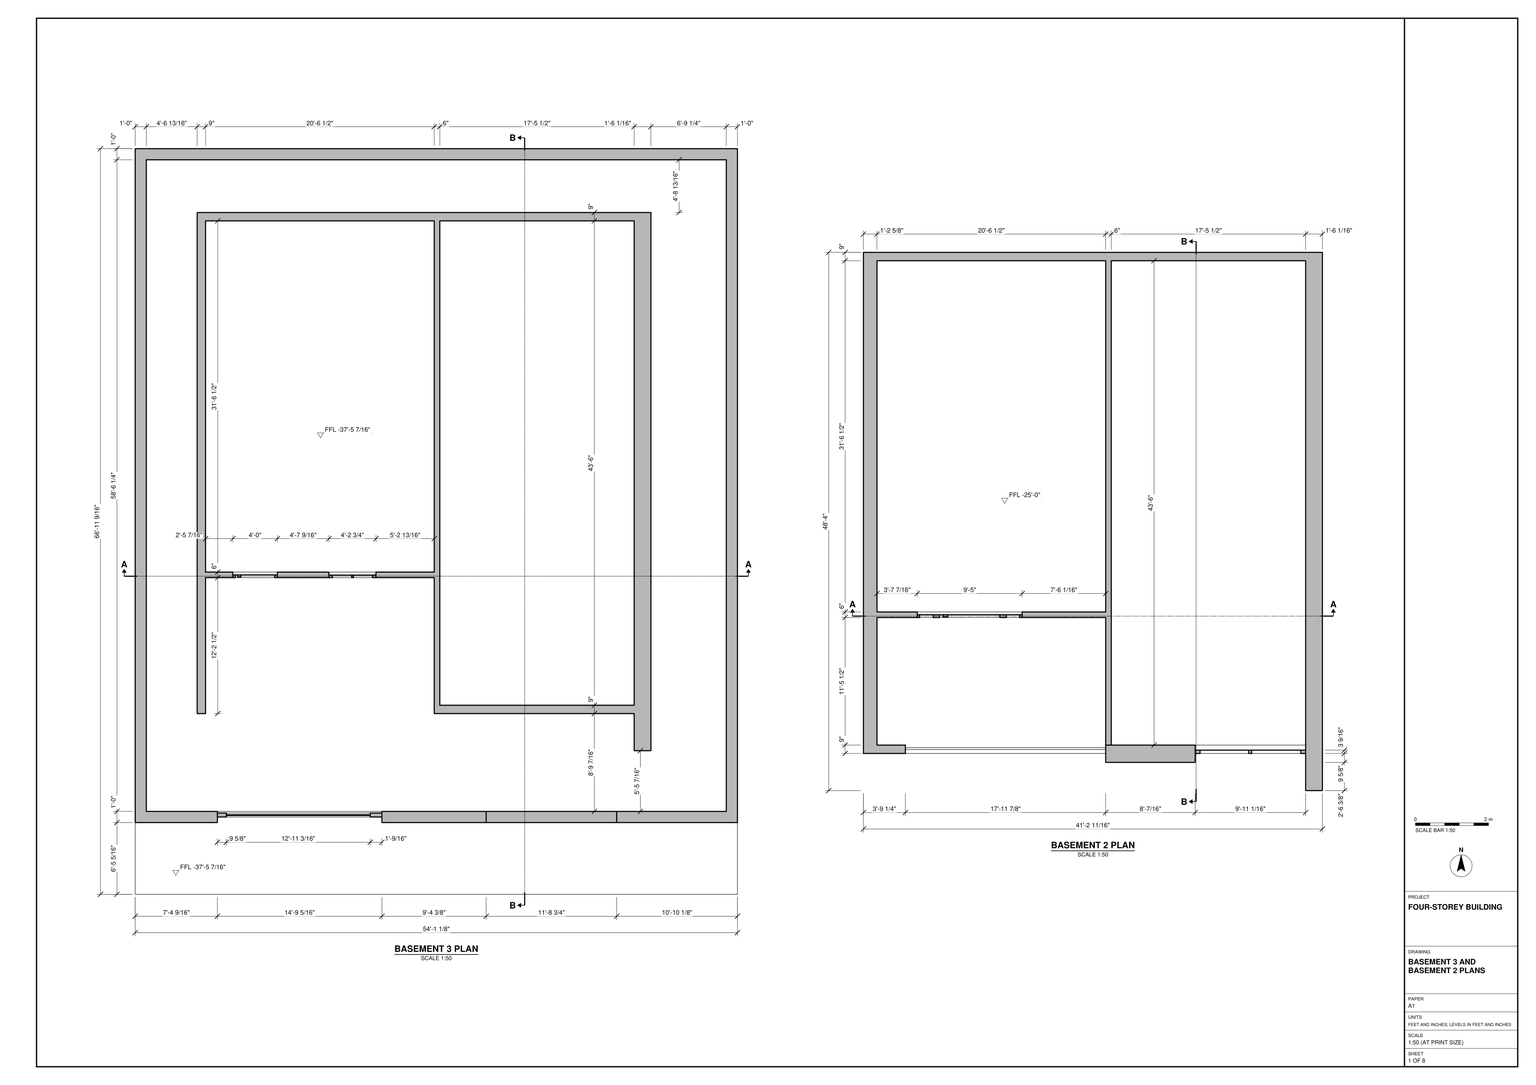
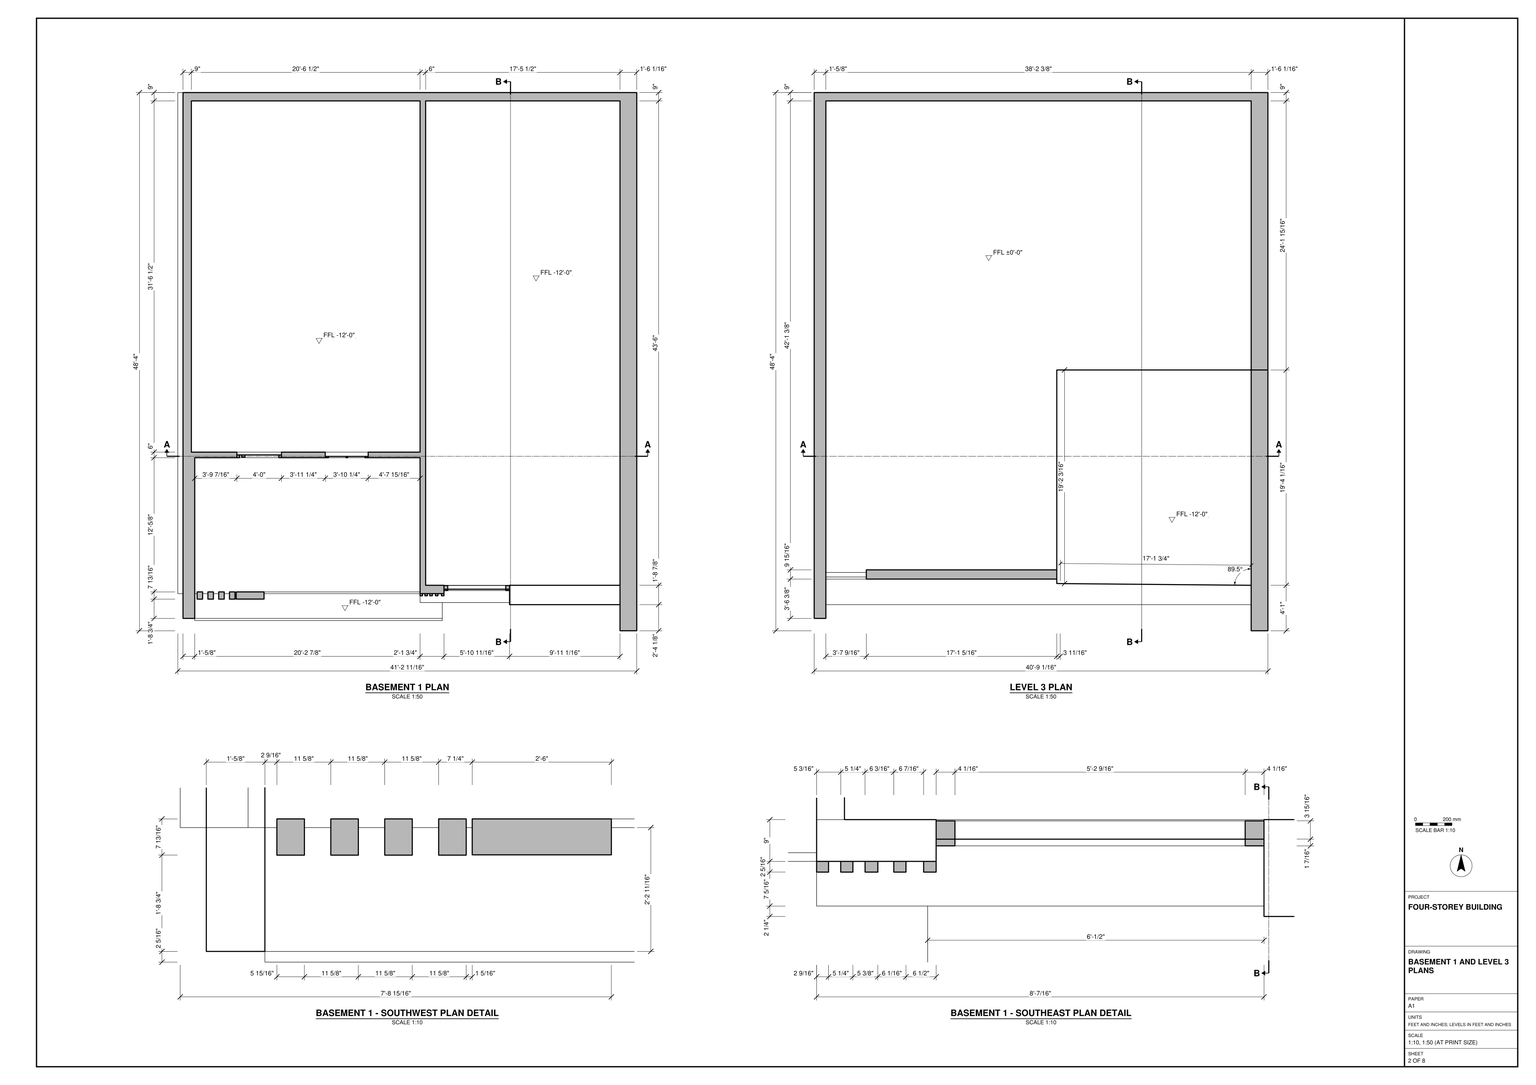
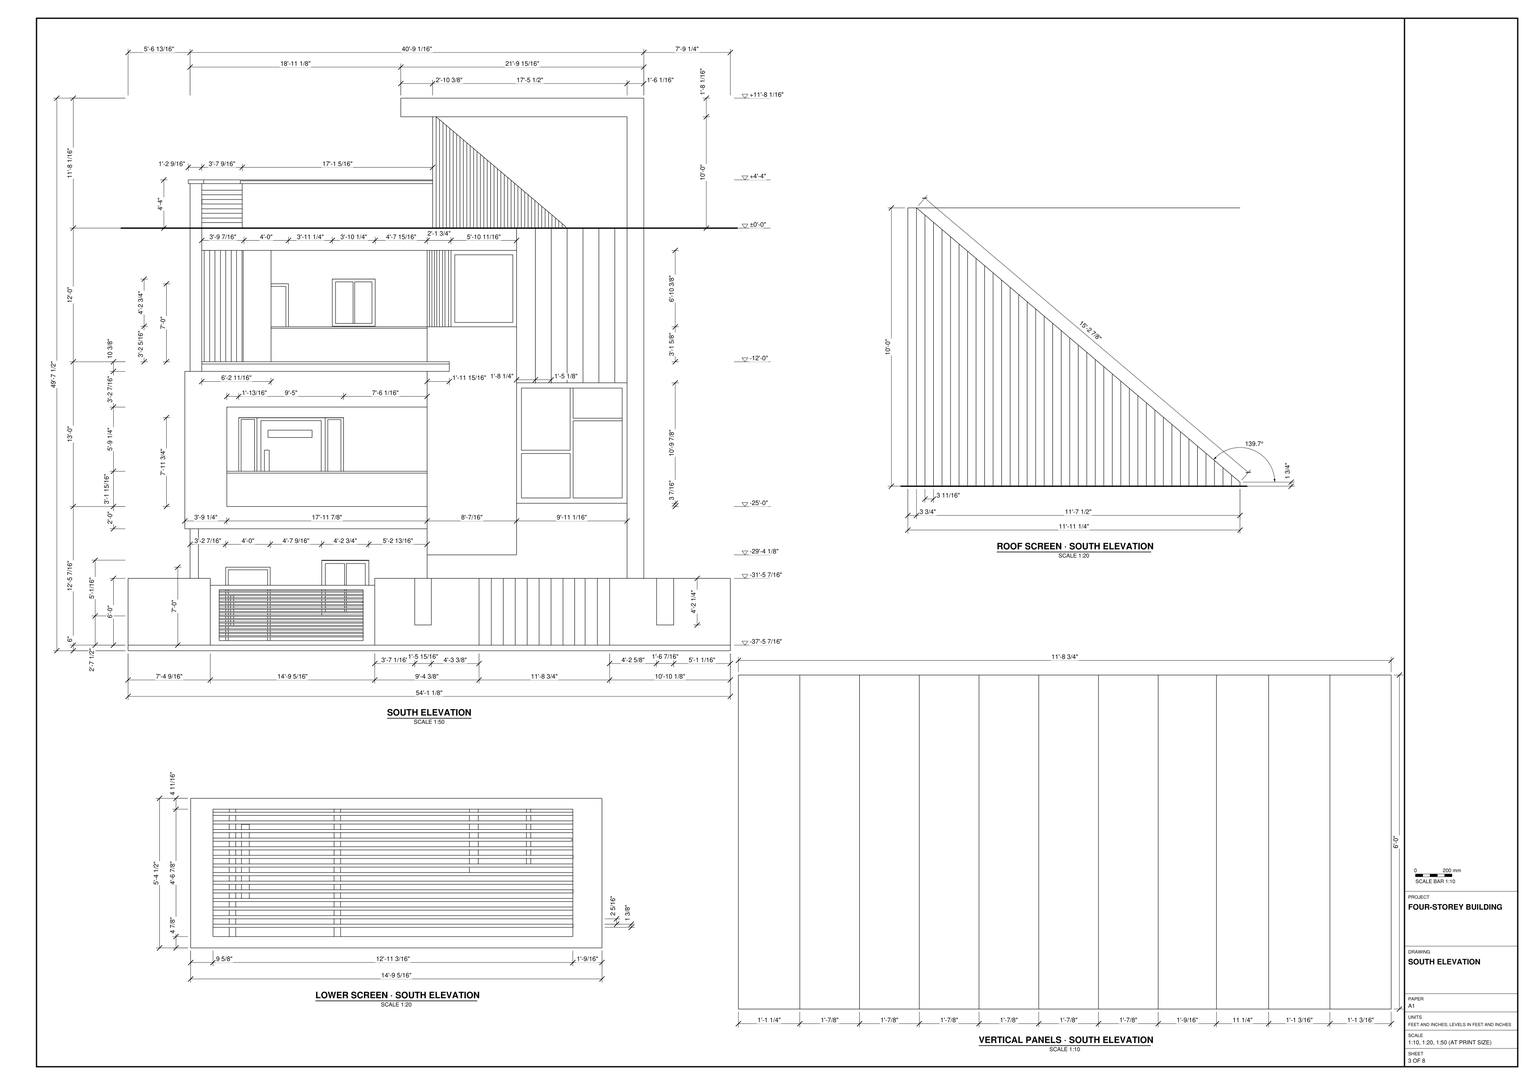
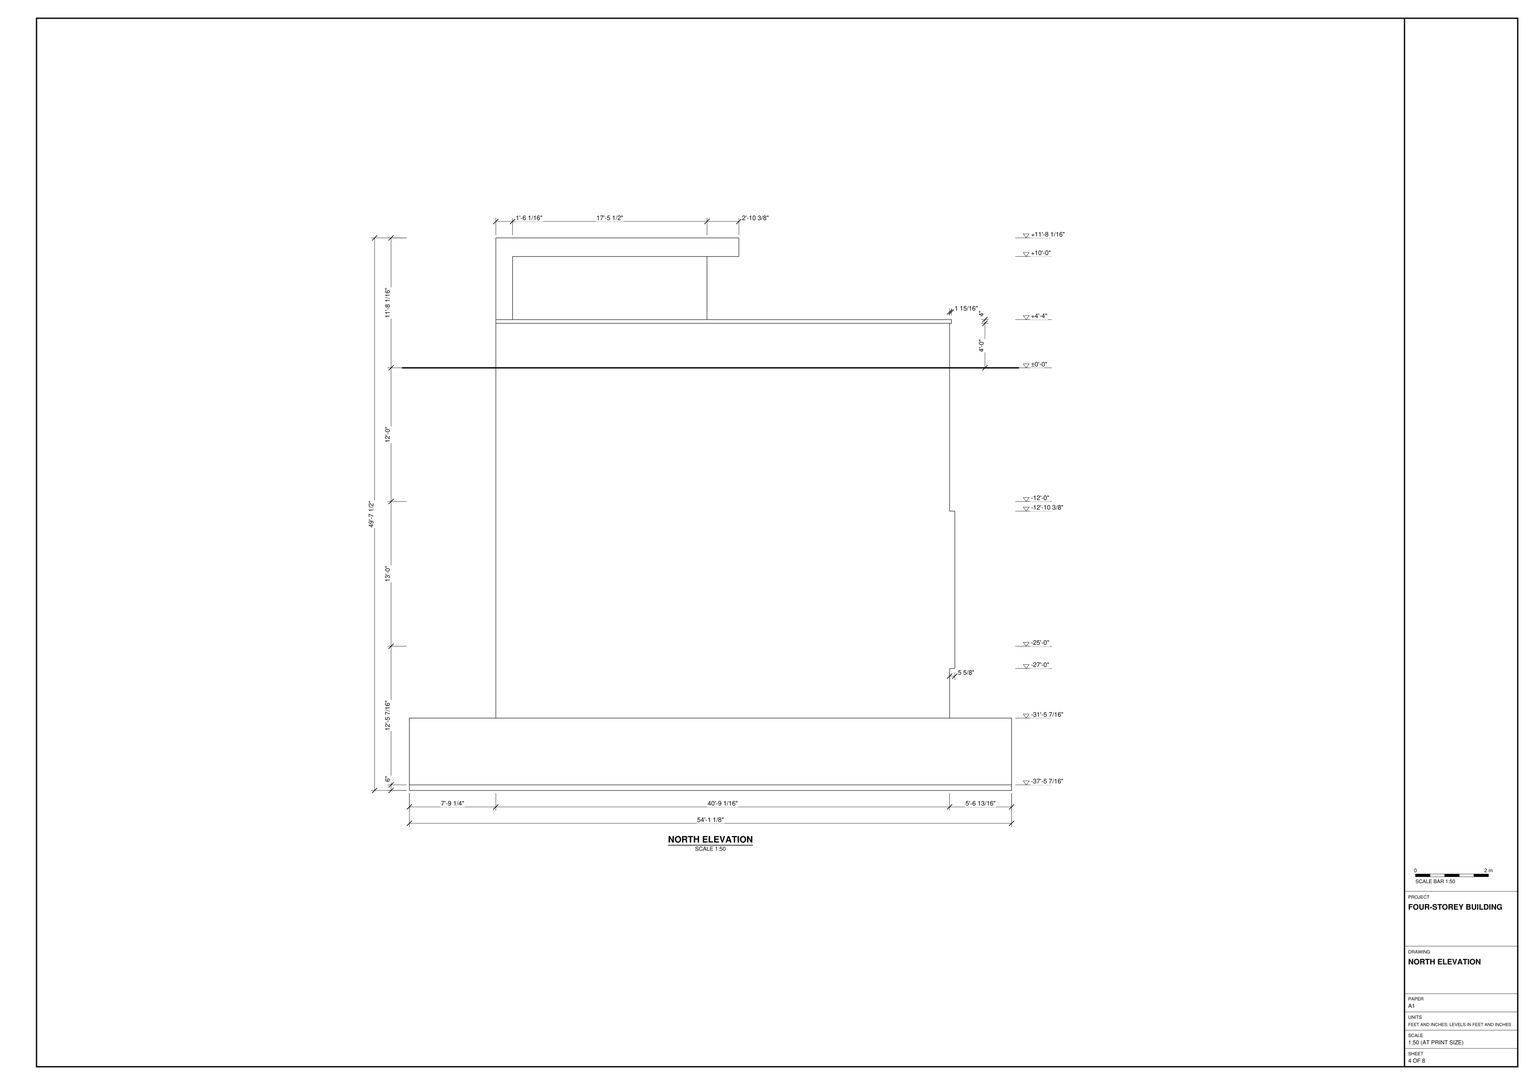
Build the four-storey building and its outer enclosure in SketchUp from task_files/diagram_01.pdf. Work in feet and inches. The complete model shall measure 69'-11 9/16" along X, 76'-9 9/16" along Y and 49'-7 1/2" along Z. Set the upper floor at ±0'-0", Basement 1 at -12'-0", Basement 2 at -25'-0" and Basement 3 at -37'-5 7/16".

Use the plans to lay out the slabs, perimeter walls and internal partitions, following the wall thicknesses and opening positions shown. Distinguish the outer enclosure at Basement 3 from the building walls inside it. Align the basement bays vertically, but follow each plan separately at the south edge, where the slab projections and recesses differ. At the upper level, preserve the southeast cutback overlooking Basement 1. Follow the sheets for stairs, built-in joinery and main furniture wherever shown.

Use the south elevation and enlarged details to model the doors, framed windows, horizontal lower screen, vertical panels and sloping roof screen beneath the raised roof frame. Decor and loose items shown may be any suitable library components. Keep shell elements such as walls, slabs and roof, and each furniture or joinery piece, in separate groups or components; use components for repeated parts. Save one SketchUp model as output_files/four_storey_building_with_a_screened_south_elevation.skp.

# SketchUp Ruby script. Lengths in inches.
U = 1.inch
M = Sketchup.active_model
def pt(a) = Geom::Point3d.new(a.map { |v| v * U })
def face(e, loops, mat)
  f = e.add_face(loops[0].map { |a| pt(a) })
  loops[1..].each { |l| e.add_face(l.map { |a| pt(a) }).erase! }
  f.material = f.back_material = mat if mat
  f
end
# faces: each face lists its corners as indices into pts; further lists are holes
def faces(e, pts, list, mat = nil) = list.each { |f| face(e, (f[0].is_a?(Array) ? f : [f]).map { |l| l.map { |i| pts[i] } }, mat) }
# xy, xz, yz: faces in a plane at the given z, y or x. An outline is a flat list of corners, or four numbers for a rectangle; further outlines are holes
def ring(l) = l.size == 4 ? [[l[0], l[1]], [l[2], l[1]], [l[2], l[3]], [l[0], l[3]]] : l.each_slice(2).to_a
def flat(e, list, mat, &to3) = list.each { |f| face(e, (f[0].is_a?(Array) ? f : [f]).map { |l| ring(l).map { |u, v| to3.(u, v) } }, mat) }
def xy(e, z, list, mat = nil) = flat(e, list, mat) { |x, y| [x, y, z] }
def xz(e, y, list, mat = nil) = flat(e, list, mat) { |x, z| [x, y, z] }
def yz(e, x, list, mat = nil) = flat(e, list, mat) { |y, z| [x, y, z] }
def lines(e, pts, list) = list.each { |a, b| e.add_line(pt(pts[a]), pt(pts[b])) }
# prism: a flat outline (further loops are holes) pulled along v
def prism(e, loops, v, mat = nil)
  f = face(e, loops, mat); d = Geom::Vector3d.new(v.map { |x| x * U })
  f.pushpull(f.normal.samedirection?(d) ? d.length : -d.length)
end
def box(e, o, s, mat = nil) = prism(e, [[o, [o[0] + s[0], o[1], o[2]], [o[0] + s[0], o[1] + s[1], o[2]], [o[0], o[1] + s[1], o[2]]]], [0, 0, s[2]], mat)
def at(x, y, z, deg = 0) = Geom::Transformation.translation(pt([x, y, z])) * Geom::Transformation.rotation(ORIGIN, Z_AXIS, deg.degrees)
def axes(o, x, y, z) = Geom::Transformation.new([*x, 0, *y, 0, *z, 0, *pt(o).to_a, 1])
def part(name) = M.definitions.add(name)
# library, detail: a bought-in or finely detailed component or shape, given as its bounding box
def library(name, o, s) = part(name).tap { |d| box(d.entities, o, s) }
def detail(e, o, s) = box(e.add_group.entities, o, s)
def put(e, d, t, mat = nil) = e.add_instance(d, t).tap { |i| i.material = mat if mat }
def group(e, t, mat = nil) = e.add_group.tap { |g| g.transformation = t; g.material = mat if mat }.entities
root = M.entities
M.materials.add("[0033_NavajoWhite]").color = [255, 222, 173]
M.materials.add("[0043_SaddleBrown]").color = [100, 69, 19]
M.materials.add("[0099_LightSteelBlue]").color = [176, 196, 222]
M.materials.add("[0134_DimGray]").color = [105, 105, 105]
M.materials.add("[Blacktop Old 01]").color = [132, 136, 139]
M.materials.add("[Color C02]").color = [255, 204, 153]
M.materials.add("[Color M04]").color = [142, 142, 142]
M.materials.add("[Color M05]").color = [114, 114, 114]
M.materials.add("[Color M06]").color = [86, 86, 86]
M.materials.add("[Concrete Aggregate Smoke]").color = [154, 150, 148]
M.materials.add("[Concrete Scored Jointless]").color = [140, 133, 127]
M.materials.add("[Metal Seamed]").color = [118, 119, 115]
M.materials.add("[Metal Silver]").color = [234, 233, 238]
M.materials.add("[Mirror 02]").color = [229, 229, 229]
M.materials.add("[Pavers with Grass Brick]").color = [187, 192, 176]
M.materials.add("[Polished Concrete Old]").color = [229, 229, 229]
M.materials.add("[Stone Brushed Khaki]").color = [226, 190, 149]
M.materials.add("[Translucent Glass Gray]").color = [128, 128, 128]
M.materials["[Translucent Glass Gray]"].alpha = 0.5
M.materials.add("[Wood Bamboo]").color = [177, 105, 43]
M.materials.add("[Wood Fence with Lattice]").color = [170, 106, 61]
M.materials.add("[Wood Floor]").color = [155, 105, 61]
c1 = part("Group\#1")
xy(c1.entities,0,[[0,0,101.9375,6.5625]],"[Wood Bamboo]")
xy(c1.entities,7.64,[[49.36,0,53.16,6.5625]])
xy(c1.entities,7.64,[[7.64,0,49.36,6.5625],[53.16,0,94.29,6.5625]],"[Wood Bamboo]")
xy(c1.entities,122.36,[[7.64,0,49.36,6.5625],[53.16,0,94.29,6.5625]],"[Wood Bamboo]")
xy(c1.entities,130,[[0,0,101.9375,6.5625]],"[Wood Bamboo]")
xz(c1.entities,0,[[[0,0,101.9375,130],[7.64,7.64,7.64,122.36,49.36,122.36,49.36,7.64,53.16,7.64,53.16,122.36,94.29,122.36,94.29,7.64]]],"[Wood Bamboo]")
xz(c1.entities,6.5625,[[7.64,7.64,49.36,122.36],[53.16,7.64,94.29,122.36]],"[Translucent Glass Gray]")
xz(c1.entities,6.5625,[[[0,0,101.9375,130],[7.64,7.64,94.29,7.64,94.29,122.36,53.16,122.36,53.16,7.64,49.36,7.64,49.36,122.36,7.64,122.36]]],"[Wood Bamboo]")
yz(c1.entities,0,[[0,0,6.5625,130]],"[Wood Bamboo]")
yz(c1.entities,7.64,[[0,7.64,6.5625,122.36]],"[Wood Bamboo]")
yz(c1.entities,49.36,[[0,7.64,6.5625,122.36]],"[Wood Bamboo]")
yz(c1.entities,53.16,[[0,7.64,6.5625,122.36]],"[Wood Bamboo]")
yz(c1.entities,94.29,[[0,7.64,6.5625,122.36]],"[Wood Bamboo]")
yz(c1.entities,101.9375,[[0,0,6.5625,130]],"[Wood Bamboo]")
c2 = part("Group\#2")
xy(c2.entities,0,[[0,0,48,3]],"[Wood Bamboo]")
xy(c2.entities,2.8,[[2.8,0,45.2,3]],"[Wood Bamboo]")
xy(c2.entities,21.03,[[5.27,0.5,8.64,3]],"[Metal Seamed]")
xy(c2.entities,53.28,[[5.27,0.5,8.64,3]],"[Metal Seamed]")
xy(c2.entities,81.2,[[2.8,0,45.2,3]],"[Wood Bamboo]")
xy(c2.entities,84,[[0,0,48,3]],"[Wood Bamboo]")
xz(c2.entities,0,[[[0,0,48,84],[2.8,2.8,45.2,81.2]]],"[Wood Bamboo]")
xz(c2.entities,0.5,[[5.27,21.03,8.64,53.28]],"[Metal Seamed]")
xz(c2.entities,3,[[[0,0,48,84],[2.8,2.8,45.2,81.2]],[[2.8,2.8,45.2,81.2],[5.27,21.03,8.64,53.28]],[5.27,21.03,8.64,53.28]],"[Wood Bamboo]")
yz(c2.entities,0,[[0,0,3,84]],"[Wood Bamboo]")
yz(c2.entities,2.8,[[0,2.8,3,81.2]],"[Wood Bamboo]")
yz(c2.entities,5.27,[[0.5,21.03,3,53.28]],"[Metal Seamed]")
yz(c2.entities,8.64,[[0.5,21.03,3,53.28]],"[Metal Seamed]")
yz(c2.entities,45.2,[[0,2.8,3,81.2]],"[Wood Bamboo]")
yz(c2.entities,48,[[0,0,3,84]],"[Wood Bamboo]")
c3 = library("Group\#3",[0,0,0],[73.75,3,84])
c4 = library("Group\#5",[0,0,0],[79.0625,3.5625,79.0625])
c5 = library("Group\#6",[0,0,0],[68.25,4.25,58.625])
xy(root,-2306.375,[[0,117.99,649.125,921.56]],"[Concrete Scored Jointless]")
xy(root,-2300.375,[[0,195.31,0,921.56,649.125,921.56,649.125,195.31,519,195.31,519,207.31,637.125,207.31,637.125,909.56,12,909.56,12,207.31,88.59,207.31,88.59,195.31],[265.91,195.31,378.28,207.31],[378.28,195.31,519,207.31],[66.8125,312.74,75.8125,459.24],[328.3125,321.74,537.8125,843.74],
  [75.8125,465.24,322.3125,843.74]])
xy(root,-2300.375,[[[12,207.31,637.125,909.56],[75.8125,465.24,322.3125,843.74],[66.8125,312.74,75.8125,459.24]]],"[Concrete Aggregate Smoke]")
xy(root,-2300.375,[[0,117.99,649.125,117.99,649.125,195.31,265.91,195.31,265.91,207.31,88.59,207.31,88.59,195.31,0,195.31]],"[Pavers with Grass Brick]")
xy(root,-2268.89,[[208.76,459.24,259.51,465.24]])
xy(root,-2228.375,[[66.8125,323.19,75.8125,459.24]],"[Color C02]")
xy(root,-2228.375,[[378.28,195.31,519,207.31]],"[Polished Concrete Old]")
xy(root,-2228.375,[[0,195.31,88.59,195.31,88.59,207.31,12,207.31,12,909.56,637.125,909.56,637.125,207.31,519,207.31,519,195.31,649.125,195.31,649.125,921.56,0,921.56],[265.91,195.31,378.28,207.31]],"[Wood Fence with Lattice]")
xy(root,-2216.375,[[105.22,459.24,153.22,465.24]])
xy(root,-2209.21,[[208.76,459.24,259.51,465.24]])
xy(root,-2203.05,[[322.3125,303.12,418.75,312.74]],"[Stone Brushed Khaki]")
xy(root,-2174.9375,[[61.1875,312.74,66.8125,323.19]])
xy(root,-2174.9375,[[61.1875,323.19,75.8125,459.24],[61.1875,459.24,66.8125,852.74]],"[Color C02]")
xy(root,-2174.9375,[[75.8125,312.74,322.3125,459.24]],"[Wood Floor]")
xy(root,-2164.25,[[75.8125,465.24,322.3125,843.74]])
xy(root,-2156.75,[[328.3125,321.74,537.8125,843.74]])
xy(root,-2150.9375,[[106.4375,316.93,322.3125,318.93],[106.4375,318.93,322.3125,318.93,322.3125,459.24,75.8125,459.24,75.8125,321.74,106.4375,321.74],[328.3125,321.74,537.8125,843.74],[119.26,459.24,232.26,465.24],[75.8125,465.24,322.3125,843.74]])
xy(root,-2150.9375,[[106.4375,312.74,322.3125,316.93]],"[Polished Concrete Old]")
xy(root,-2147.48,[[418.75,312.74,537.8125,321.74]])
xy(root,-2115,[[106.4375,316.93,322.3125,318.93]])
xy(root,-2113,[[106.4375,316.93,322.3125,318.93]],"[Metal Silver]")
xy(root,-2055.3125,[[119.26,459.24,232.26,465.24]])
xy(root,-2043.75,[[106.4375,312.74,322.3125,321.74]],"[Polished Concrete Old]")
xy(root,-2030.9375,[[75.8125,321.74,322.3125,459.24]],"[Wood Floor]")
xy(root,-2017.62,[[418.75,300.87,537.8125,321.74]])
xy(root,-2015.125,[[75.8125,465.24,322.3125,843.74]])
xy(root,-2005.3125,[[66.8125,286.06,79.4375,312.74],[322.3125,303.12,346.25,312.74]])
xy(root,-2005.3125,[[61.1875,312.74,66.8125,852.74]],"[Color C02]")
xy(root,-2005.3125,[[79.4375,286.06,79.4375,312.74,322.3125,312.74,322.3125,303.12,346.25,303.12,346.25,286.06]],"[Color M05]")
xy(root,-1999,[[328.3125,321.74,537.8125,843.74]])
xy(root,-1997.375,[[79.4375,286.06,346.25,312.74]])
xy(root,-1997.375,[[79.4375,283.74,346.25,286.06]],"[Color M05]")
xy(root,-1994.9375,[[322.3125,303.12,346.25,312.74],[82.02,306.81,87.96,312.74],[93.65,306.81,99.58,312.74],[105.27,306.81,111.21,312.74],[116.9,306.81,122.83,312.74],
  [124.125,306.87,154.125,312.74],[75.8125,312.74,79.4375,459.24],[82.02,312.74,87.96,314.62],[93.65,312.74,99.58,314.62],[105.27,312.74,111.21,314.62],
  [116.9,312.74,122.83,314.62],[124.125,312.74,154.125,314.62],[154.125,312.74,322.3125,314.62],[328.3125,321.74,537.8125,843.74],[124.9,459.24,172.9,465.24],
  [75.8125,465.24,322.3125,843.74]])
xy(root,-1994.9375,[[79.4375,283.74,346.25,286.06],[79.4375,312.74,82.02,312.74,82.02,314.62,87.96,314.62,87.96,312.74,93.65,312.74,93.65,314.62,99.58,314.62,99.58,312.74,105.27,312.74,105.27,314.62,111.21,314.62,111.21,312.74,116.9,312.74,116.9,314.62,122.83,314.62,122.83,312.74,124.125,312.74,124.125,314.62,322.3125,314.62,322.3125,459.24,79.4375,459.24]],"[Color M05]")
xy(root,-1994.9375,[[79.4375,286.06,346.25,286.06,346.25,303.12,322.3125,303.12,322.3125,312.74,154.125,312.74,154.125,306.87,124.125,306.87,124.125,312.74,122.83,312.74,122.83,306.81,116.9,306.81,116.9,312.74,111.21,312.74,111.21,306.81,105.27,306.81,105.27,312.74,99.58,312.74,99.58,306.81,93.65,306.81,93.65,312.74,87.96,312.74,87.96,306.81,82.02,306.81,82.02,312.74,79.4375,312.74]],"[Color M06]")
xy(root,-1958.9375,[[154.125,312.74,322.3125,314.62]])
xy(root,-1957.3125,[[322.3125,310.43,324.88,312.74],[327.51,310.43,330.13,312.74],[332.76,310.43,335.51,312.74],[338.95,310.43,341.57,312.74],[345.38,310.43,348.07,312.74]])
xy(root,-1957.3125,[[154.125,312.74,322.3125,314.62]],"[Metal Silver]")
xy(root,-1957.3125,[[322.3125,303.12,418.75,303.12,418.75,321.74,348.07,321.74,348.07,310.43,345.38,310.43,345.38,312.74,341.57,312.74,341.57,310.43,338.95,310.43,338.95,312.74,335.51,312.74,335.51,310.43,332.76,310.43,332.76,312.74,330.13,312.74,330.13,310.43,327.51,310.43,327.51,312.74,324.88,312.74,324.88,310.43,322.3125,310.43]],"[Stone Brushed Khaki]")
xy(root,-1956.62,[[220.125,459.24,266.375,465.24]])
xy(root,-1910.9375,[[124.9,459.24,172.9,465.24]])
xy(root,-1905.81,[[220.125,459.24,266.375,465.24]])
xy(root,-1875,[[82.02,306.81,87.96,314.62]])
xy(root,-1874.9375,[[322.3125,300.87,322.3125,310.43,324.88,310.43,324.88,312.74,327.51,312.74,327.51,310.43,330.13,310.43,330.13,312.74,332.76,312.74,332.76,310.43,335.51,310.43,335.51,312.74,338.95,312.74,338.95,310.43,341.57,310.43,341.57,312.74,345.38,312.74,345.38,310.43,348.07,310.43,348.07,321.74,418.75,321.74,418.75,300.87],[322.3125,310.43,324.88,312.74],[327.51,310.43,330.13,312.74],[332.76,310.43,335.51,312.74],[338.95,310.43,341.57,312.74],
  [345.38,310.43,348.07,312.74]])
xy(root,-1874.9375,[[[79.4375,300.87,322.3125,459.24],[124.125,306.87,154.125,314.62],[93.65,306.81,99.58,314.62],[105.27,306.81,111.21,314.62],[116.9,306.81,122.83,314.62]]],"[Wood Floor]")
xy(root,-1857.1875,[[328.3125,321.74,537.8125,843.74]])
xy(root,-1856.8125,[[75.8125,465.24,322.3125,843.74]])
xy(root,-1850.9375,[[537.8125,321.74,471.54,322.34,464.2,322.41,460.52,322.44,456.85,322.47,453.18,322.51,445.84,322.57,442.17,322.61,434.83,322.67,431.16,322.71,423.82,322.77,420.14,322.81,412.8,322.87,409.13,322.91,405.46,322.9375,401.79,322.97,398.12,323,394.45,323.04,387.11,323.1,383.4375,323.14,379.76,323.17,376.09,323.2,372.42,323.24,365.08,323.3,361.41,323.34,354.07,323.4,350.4,323.4375,346.73,323.47,343.06,323.5,339.38,323.54,332.04,323.6,328.3125,323.66,328.3125,553.79,537.8125,553.79],[123.02,328.43,328.3125,338.37],[537.8125,553.79,555.875,852.74],[79.4375,843.74,537.8125,852.74]])
xy(root,-1850.9375,[[79.4375,300.87,537.8125,300.87,537.8125,321.74,471.54,322.34,464.2,322.41,460.52,322.44,456.85,322.47,453.18,322.51,445.84,322.57,442.17,322.61,434.83,322.67,431.16,322.71,423.82,322.77,420.14,322.81,412.8,322.87,409.13,322.91,405.46,322.9375,401.79,322.97,398.12,323,394.45,323.04,387.11,323.1,383.4375,323.14,379.76,323.17,376.09,323.2,372.42,323.24,365.08,323.3,361.41,323.34,354.07,323.4,350.4,323.4375,346.73,323.47,343.06,323.5,339.38,323.54,332.04,323.6,328.3125,323.66,328.3125,328.43,79.4375,328.43]],"[0099_LightSteelBlue]")
xy(root,-1850.9375,[[79.4375,328.43,123.02,328.43,123.02,338.37,328.3125,338.37,328.3125,553.79,537.8125,553.79,537.8125,843.74,79.4375,843.74]],"[Blacktop Old 01]")
xy(root,-1844.98,[[123.02,330.7,148.02,335.57]])
xy(root,-1844.98,[[79.4375,330.7,123.02,335.57]],"[Color M05]")
xy(root,-1840.1,[[123.02,330.7,148.02,335.57]])
xy(root,-1840.1,[[79.4375,330.7,123.02,335.57]],"[Color M05]")
xy(root,-1834.98,[[123.02,330.7,148.02,335.57]])
xy(root,-1834.98,[[79.4375,330.7,123.02,335.57]],"[Color M05]")
xy(root,-1830.1,[[123.02,330.7,148.02,335.57]])
xy(root,-1830.1,[[79.4375,330.7,123.02,335.57]],"[Color M05]")
xy(root,-1824.98,[[123.02,330.7,148.02,335.57]])
xy(root,-1824.98,[[79.64,330.7,123.02,335.57]],"[Color M05]")
xy(root,-1820.1,[[123.02,330.7,148.02,335.57]])
xy(root,-1820.1,[[79.64,330.7,123.02,335.57]],"[Color M05]")
xy(root,-1814.98,[[123.02,330.7,148.02,335.57]])
xy(root,-1814.98,[[79.4375,330.7,123.02,335.57]],"[Color M05]")
xy(root,-1810.1,[[123.02,330.7,148.02,335.57]])
xy(root,-1810.1,[[79.4375,330.7,123.02,335.57]],"[Color M05]")
xy(root,-1802.9375,[[64.875,279.87,64.875,852.74,66.8125,852.74,66.8125,286.06,79.4375,286.06,79.4375,843.74,81.5,843.74,81.5,279.87],[66.8125,286.06,79.4375,852.74],[123.02,328.43,123.02,330.7,148.02,330.7,148.02,335.57,123.02,335.57,123.02,338.37,328.3125,338.37,328.3125,328.43],[123.02,330.7,148.02,335.57],[537.8125,553.79,555.875,852.74],
  [79.4375,843.74,81.5,852.74],[81.5,843.74,537.8125,852.74]])
xy(root,-1802.9375,[[120.95,327.24,120.95,339.56,328.3125,339.56,328.3125,338.37,123.02,338.37,123.02,328.43,328.3125,328.43,328.3125,327.24]],"[Color M05]")
xy(root,-1799.9375,[[120.95,327.24,328.3125,339.56]],"[Color M05]")
xy(root,-1798.9375,[[64.875,279.87,81.5,279.87,81.5,843.74,537.8125,843.74,537.8125,553.79,555.875,553.79,555.875,852.74,64.875,852.74]],"[Color M04]")
xy(root,-1730.9375,[[293.9375,272.74,293.9375,553.79,328.3125,553.79,328.3125,323.66,332.04,323.6,537.8125,321.74,537.8125,272.74],[537.8125,321.74,332.04,323.6,328.3125,323.66,328.3125,553.79,537.8125,553.79]])
xy(root,-1710.875,[[293.9375,272.74,555.875,553.79]])
xz(root,117.99,[[0,-2306.375,649.125,-2300.375]],"[Concrete Scored Jointless]")
xz(root,195.31,[[308.96,-2278.625,326.9,-2228.375],[569.63,-2278.625,588.06,-2228.375]],"[0134_DimGray]")
xz(root,195.31,[[378.28,-2300.375,391.53,-2228.375],[391.53,-2300.375,404.4,-2228.375],[404.4,-2300.375,417.28,-2228.375],[417.28,-2300.375,430.15,-2228.375],[430.15,-2300.375,443.03,-2228.375],
  [443.03,-2300.375,455.9,-2228.375],[455.9,-2300.375,468.78,-2228.375],[468.78,-2300.375,481.34,-2228.375],[481.34,-2300.375,492.59,-2228.375],[492.59,-2300.375,505.8,-2228.375],
  [505.8,-2300.375,519,-2228.375]],"[Polished Concrete Old]")
xz(root,195.31,[[0,-2300.375,88.59,-2228.375],[265.91,-2300.375,378.28,-2300.375,378.28,-2228.375,326.9,-2228.375,326.9,-2278.625,308.96,-2278.625,308.96,-2228.375,265.91,-2228.375],[519,-2300.375,649.125,-2300.375,649.125,-2228.375,588.06,-2228.375,588.06,-2278.625,569.63,-2278.625,569.63,-2228.375,519,-2228.375]],"[Wood Fence with Lattice]")
xz(root,207.31,[[378.28,-2300.375,519,-2228.375]],"[Polished Concrete Old]")
xz(root,207.31,[[12,-2300.375,88.59,-2228.375],[265.91,-2300.375,378.28,-2228.375],[519,-2300.375,637.125,-2228.375]],"[Wood Fence with Lattice]")
xz(root,272.74,[[537.8125,-2300.375,555.875,-2300.375,555.875,-1710.875,293.9375,-1710.875,293.9375,-1730.9375,537.8125,-1730.9375]])
xz(root,279.87,[[64.875,-1802.9375,81.5,-1798.9375]],"[Color M04]")
xz(root,283.74,[[79.4375,-1997.375,346.25,-1994.9375]],"[Color M05]")
xz(root,286.06,[[79.4375,-1997.375,346.25,-1994.9375]])
xz(root,286.06,[[66.8125,-2005.3125,79.4375,-1802.9375]],"[0099_LightSteelBlue]")
xz(root,286.06,[[79.4375,-2005.3125,346.25,-1997.375]],"[Color M05]")
xz(root,300.87,[[418.75,-2017.62,438.97,-1850.9375],[438.97,-2017.62,456.1,-1850.9375],[456.1,-2017.62,473.22,-1850.9375],[473.22,-2017.62,490.35,-1850.9375],[490.35,-2017.62,507.47,-1850.9375],
  [507.47,-2017.62,524.6,-1850.9375],[524.6,-2017.62,537.8125,-1850.9375],[79.4375,-1874.9375,418.75,-1850.9375]],"[0099_LightSteelBlue]")
xz(root,303.12,[[322.3125,-2203.05,418.75,-2203.05,418.75,-1957.3125,322.3125,-1957.3125,322.3125,-1994.9375,346.25,-1994.9375,346.25,-2005.3125,322.3125,-2005.3125]],"[Stone Brushed Khaki]")
xz(root,306.81,[[82.02,-1994.9375,87.96,-1875],[93.65,-1994.9375,99.58,-1874.9375],[105.27,-1994.9375,111.21,-1874.9375],[116.9,-1994.9375,122.83,-1874.9375]],"[Color M05]")
xz(root,306.87,[[124.125,-1994.9375,154.125,-1874.9375]],"[Color M05]")
xz(root,310.43,[[322.3125,-1957.3125,324.88,-1874.9375],[327.51,-1957.3125,330.13,-1874.9375],[332.76,-1957.3125,335.51,-1874.9375],[338.95,-1957.3125,341.57,-1874.9375],[345.38,-1957.3125,348.07,-1874.9375]],"[Wood Floor]")
xz(root,312.74,[[75.8125,-2005.3125,79.4375,-1994.9375],[79.4375,-2005.3125,322.3125,-1997.375],[322.3125,-2005.3125,346.25,-1997.375],[79.4375,-1997.375,322.3125,-1994.9375],[322.3125,-1997.375,346.25,-1994.9375],
  [322.3125,-1957.3125,324.88,-1874.9375],[327.51,-1957.3125,330.13,-1874.9375],[332.76,-1957.3125,335.51,-1874.9375],[338.95,-1957.3125,341.57,-1874.9375],[345.38,-1957.3125,348.07,-1874.9375]])
xz(root,312.74,[[66.8125,-2300.375,75.8125,-2174.9375]],"[Color C02]")
xz(root,312.74,[[154.125,-1958.9375,322.3125,-1957.3125]],"[Metal Silver]")
xz(root,312.74,[[322.3125,-2300.375,537.8125,-2300.375,537.8125,-2147.48,418.75,-2147.48,418.75,-2203.05,322.3125,-2203.05],[61.1875,-2174.9375,322.3125,-2174.9375,322.3125,-2150.9375,106.4375,-2150.9375,106.4375,-2043.75,322.3125,-2043.75,322.3125,-2005.3125,61.1875,-2005.3125]],"[Polished Concrete Old]")
xz(root,312.74,[[154.125,-1994.9375,322.3125,-1958.9375]],"[Translucent Glass Gray]")
xz(root,312.74,[[324.88,-1957.3125,327.51,-1874.9375],[330.13,-1957.3125,332.76,-1874.9375],[335.51,-1957.3125,338.95,-1874.9375],[341.57,-1957.3125,345.38,-1874.9375]],"[Wood Floor]")
xz(root,314.62,[[82.02,-1994.9375,87.96,-1875],[93.65,-1994.9375,99.58,-1874.9375],[105.27,-1994.9375,111.21,-1874.9375],[116.9,-1994.9375,122.83,-1874.9375],[124.125,-1994.9375,154.125,-1874.9375]],"[Color M05]")
xz(root,314.62,[[154.125,-1958.9375,322.3125,-1957.3125]],"[Metal Silver]")
xz(root,314.62,[[154.125,-1994.9375,322.3125,-1958.9375]],"[Translucent Glass Gray]")
xz(root,316.93,[[106.4375,-2115,322.3125,-2113]],"[Metal Silver]")
xz(root,316.93,[[106.4375,-2150.9375,322.3125,-2115]],"[Translucent Glass Gray]")
xz(root,318.93,[[106.4375,-2115,322.3125,-2113]],"[Metal Silver]")
xz(root,318.93,[[106.4375,-2150.9375,322.3125,-2115]],"[Wood Fence with Lattice]")
xz(root,321.74,[[328.3125,-2300.375,537.8125,-2156.75],[322.3125,-2174.9375,328.3125,-2150.9375],[328.3125,-2156.75,362.57,-2150.9375],[362.57,-2156.75,372.26,-2150.9375],[372.26,-2156.75,537.8125,-2150.9375],
  [75.8125,-2150.9375,106.4375,-2043.75],[322.3125,-2150.9375,328.3125,-2030.9375],[328.3125,-2150.9375,328.3125,-1999,537.8125,-1999,537.8125,-2017.62,418.75,-2017.62,418.75,-2147.48,537.8125,-2147.48,537.8125,-2150.9375],[75.8125,-2043.75,322.3125,-2030.9375],[322.3125,-2030.9375,328.3125,-1994.9375],
  [328.3125,-1999,537.8125,-1994.9375],[328.3125,-1994.9375,328.3125,-1874.9375,348.07,-1874.9375,348.07,-1957.3125,418.75,-1957.3125,418.75,-1874.9375,537.8125,-1874.9375,537.8125,-1994.9375],[328.3125,-1874.9375,537.8125,-1857.1875]])
xz(root,323.19,[[66.8125,-2228.375,75.8125,-2174.9375]],"[Color C02]")
xz(root,327.24,[[120.95,-1802.9375,328.3125,-1799.9375]],"[Color M05]")
xz(root,328.43,[[123.02,-1850.9375,328.3125,-1802.9375]],"[Color M05]")
xz(root,330.7,[[123.02,-1844.98,148.02,-1840.1],[123.02,-1834.98,148.02,-1830.1],[123.02,-1824.98,148.02,-1820.1],[123.02,-1814.98,148.02,-1810.1]])
xz(root,330.7,[[79.4375,-1844.98,123.02,-1840.1],[79.4375,-1834.98,123.02,-1830.1],[79.64,-1824.98,123.02,-1820.1],[79.4375,-1814.98,123.02,-1810.1]],"[Color M05]")
xz(root,335.57,[[123.02,-1844.98,148.02,-1840.1],[123.02,-1834.98,148.02,-1830.1],[123.02,-1824.98,148.02,-1820.1],[123.02,-1814.98,148.02,-1810.1]])
xz(root,335.57,[[79.4375,-1844.98,123.02,-1840.1],[79.4375,-1834.98,123.02,-1830.1],[79.64,-1824.98,123.02,-1820.1],[79.4375,-1814.98,123.02,-1810.1]],"[Color M05]")
xz(root,338.37,[[123.02,-1850.9375,328.3125,-1802.9375]],"[Color M05]")
xz(root,339.56,[[120.95,-1802.9375,328.3125,-1799.9375]],"[Color M05]")
xz(root,459.24,[[75.8125,-2174.9375,322.3125,-2150.9375],[75.8125,-2030.9375,322.3125,-1994.9375]])
xz(root,459.24,[[[75.8125,-2300.375,105.22,-2300.375,105.22,-2216.375,153.22,-2216.375,153.22,-2300.375,322.3125,-2300.375,322.3125,-2174.9375,75.8125,-2174.9375],[208.76,-2268.89,259.51,-2209.21]],[[79.4375,-1994.9375,124.9,-1994.9375,124.9,-1910.9375,172.9,-1910.9375,172.9,-1994.9375,322.3125,-1994.9375,322.3125,-1874.9375,79.4375,-1874.9375],[220.125,-1956.62,266.375,-1905.81]]],"[0033_NavajoWhite]")
xz(root,459.24,[[66.8125,-2228.375,75.8125,-2174.9375],[75.8125,-2150.9375,119.26,-2150.9375,119.26,-2055.3125,232.26,-2055.3125,232.26,-2150.9375,322.3125,-2150.9375,322.3125,-2030.9375,75.8125,-2030.9375]],"[Color C02]")
xz(root,465.24,[[[75.8125,-2300.375,75.8125,-2174.9375,322.3125,-2174.9375,322.3125,-2300.375,153.22,-2300.375,153.22,-2216.375,105.22,-2216.375,105.22,-2300.375],[208.76,-2268.89,259.51,-2209.21]],[75.8125,-2174.9375,322.3125,-2164.25],[75.8125,-2164.25,119.26,-2150.9375],[119.26,-2164.25,232.26,-2150.9375],[232.26,-2164.25,322.3125,-2150.9375],
  [75.8125,-2150.9375,75.8125,-2030.9375,322.3125,-2030.9375,322.3125,-2150.9375,232.26,-2150.9375,232.26,-2055.3125,119.26,-2055.3125,119.26,-2150.9375],[75.8125,-2030.9375,322.3125,-2015.125],[75.8125,-2015.125,124.9,-1994.9375],[124.9,-2015.125,172.9,-1994.9375],[172.9,-2015.125,322.3125,-1994.9375],
  [[75.8125,-1994.9375,75.8125,-1874.9375,322.3125,-1874.9375,322.3125,-1994.9375,172.9,-1994.9375,172.9,-1910.9375,124.9,-1910.9375,124.9,-1994.9375],[220.125,-1956.62,266.375,-1905.81]],[75.8125,-1874.9375,322.3125,-1856.8125]])
xz(root,553.79,[[537.8125,-1850.9375,555.875,-1802.9375],[537.8125,-1802.9375,555.875,-1798.9375],[537.8125,-1798.9375,537.8125,-1730.9375,293.9375,-1730.9375,293.9375,-1710.875,555.875,-1710.875,555.875,-1798.9375]])
xz(root,553.79,[[328.3125,-1850.9375,537.8125,-1730.9375]],"[Wood Floor]")
xz(root,843.74,[[75.8125,-2300.375,322.3125,-2164.25],[328.3125,-2300.375,537.8125,-2174.9375],[328.3125,-2174.9375,537.8125,-2156.75],[75.8125,-2164.25,93.4375,-2150.9375],[93.4375,-2164.25,322.3125,-2150.9375],
  [328.3125,-2156.75,537.8125,-2150.9375],[75.8125,-2150.9375,322.3125,-2015.125],[328.3125,-2150.9375,537.8125,-2030.9375],[328.3125,-2030.9375,537.8125,-1999],[75.8125,-2015.125,85.59,-1994.9375],
  [85.59,-2015.125,95.84,-1994.9375],[95.84,-2015.125,322.3125,-1994.9375],[328.3125,-1999,537.8125,-1994.9375],[75.8125,-1994.9375,322.3125,-1856.8125],[328.3125,-1994.9375,537.8125,-1857.1875],
  [328.3125,-1857.1875,537.8125,-1850.9375],[88.0625,-1856.8125,322.3125,-1850.9375]])
xz(root,843.74,[[79.4375,-1850.9375,537.8125,-1802.9375],[81.5,-1802.9375,537.8125,-1798.9375]],"[Color M04]")
xz(root,852.74,[[66.8125,-2300.375,66.8125,-2174.9375,61.1875,-2174.9375,61.1875,-2005.3125,66.8125,-2005.3125,66.8125,-1850.9375,555.875,-1850.9375,555.875,-2300.375]],"[Color C02]")
xz(root,852.74,[[66.8125,-1850.9375,555.875,-1802.9375],[64.875,-1802.9375,555.875,-1798.9375]],"[Color M04]")
xz(root,909.56,[[12,-2300.375,637.125,-2228.375]],"[Wood Fence with Lattice]")
xz(root,921.56,[[0,-2306.375,649.125,-2300.375]],"[Concrete Scored Jointless]")
xz(root,921.56,[[0,-2300.375,649.125,-2228.375]],"[Wood Fence with Lattice]")
yz(root,0,[[117.99,-2306.375,921.56,-2300.375]],"[Concrete Scored Jointless]")
yz(root,0,[[195.31,-2300.375,921.56,-2228.375]],"[Wood Fence with Lattice]")
yz(root,12,[[207.31,-2300.375,909.56,-2228.375]],"[Wood Fence with Lattice]")
yz(root,61.1875,[[312.74,-2174.9375,852.74,-2005.3125]],"[Color C02]")
yz(root,64.875,[[279.87,-1802.9375,852.74,-1798.9375]],"[Color M04]")
yz(root,66.8125,[[312.74,-2300.375,312.74,-2174.9375,323.19,-2174.9375,323.19,-2228.375,459.24,-2228.375,459.24,-2174.9375,852.74,-2174.9375,852.74,-2300.375],[286.06,-2005.3125,852.74,-1850.9375]],"[Color C02]")
yz(root,66.8125,[[286.06,-1850.9375,852.74,-1802.9375]],"[Color M04]")
yz(root,75.8125,[[465.24,-2300.375,843.74,-2164.25],[321.74,-2174.9375,459.24,-2150.9375],[465.24,-2164.25,843.74,-2150.9375],[465.24,-2150.9375,843.74,-2015.125],[465.24,-2015.125,843.74,-1994.9375],
  [465.24,-1994.9375,843.74,-1856.8125]])
yz(root,75.8125,[[312.74,-2300.375,459.24,-2300.375,459.24,-2228.375,323.19,-2228.375,323.19,-2174.9375,312.74,-2174.9375],[321.74,-2150.9375,459.24,-2030.9375]],"[0033_NavajoWhite]")
yz(root,79.4375,[[286.06,-2005.3125,312.74,-1997.375],[286.06,-1997.375,312.74,-1994.9375],[300.87,-1874.9375,459.24,-1850.9375]])
yz(root,79.4375,[[[286.06,-1994.9375,459.24,-1994.9375,459.24,-1874.9375,300.87,-1874.9375,300.87,-1850.9375,843.74,-1850.9375,843.74,-1802.9375,286.06,-1802.9375],[330.7,-1814.98,335.57,-1810.1],[330.7,-1834.98,335.57,-1830.1],[330.7,-1844.98,335.57,-1840.1]]],"[0099_LightSteelBlue]")
yz(root,79.4375,[[283.74,-1997.375,286.06,-1994.9375]],"[Color M05]")
yz(root,79.64,[[330.7,-1824.98,335.57,-1820.1]])
yz(root,81.5,[[279.87,-1802.9375,843.74,-1798.9375]],"[Color M04]")
yz(root,82.02,[[306.81,-1994.9375,314.62,-1875]],"[Color M05]")
yz(root,87.96,[[306.81,-1994.9375,314.62,-1875]],"[Color M05]")
yz(root,88.59,[[195.31,-2300.375,207.31,-2228.375]],"[Wood Fence with Lattice]")
yz(root,93.65,[[306.81,-1994.9375,314.62,-1874.9375]],"[Color M05]")
yz(root,99.58,[[306.81,-1994.9375,314.62,-1874.9375]],"[Color M05]")
yz(root,105.22,[[459.24,-2300.375,465.24,-2216.375]])
yz(root,105.27,[[306.81,-1994.9375,314.62,-1874.9375]],"[Color M05]")
yz(root,106.4375,[[316.93,-2150.9375,318.93,-2115],[316.93,-2115,318.93,-2113]])
yz(root,106.4375,[[312.74,-2150.9375,316.93,-2150.9375,316.93,-2113,318.93,-2113,318.93,-2150.9375,321.74,-2150.9375,321.74,-2043.75,312.74,-2043.75]],"[Polished Concrete Old]")
yz(root,111.21,[[306.81,-1994.9375,314.62,-1874.9375]],"[Color M05]")
yz(root,116.9,[[306.81,-1994.9375,314.62,-1874.9375]],"[Color M05]")
yz(root,119.26,[[459.24,-2150.9375,465.24,-2055.3125]])
yz(root,120.95,[[327.24,-1802.9375,339.56,-1799.9375]],"[Color M05]")
yz(root,122.83,[[306.81,-1994.9375,314.62,-1874.9375]],"[Color M05]")
yz(root,123.02,[[[328.43,-1850.9375,338.37,-1802.9375],[330.7,-1844.98,335.57,-1840.1],[330.7,-1834.98,335.57,-1830.1],[330.7,-1824.98,335.57,-1820.1],[330.7,-1814.98,335.57,-1810.1]]],"[Color M05]")
yz(root,124.125,[[306.87,-1994.9375,314.62,-1874.9375]],"[Color M05]")
yz(root,124.9,[[459.24,-1994.9375,465.24,-1910.9375]])
yz(root,148.02,[[330.7,-1844.98,335.57,-1840.1],[330.7,-1834.98,335.57,-1830.1],[330.7,-1824.98,335.57,-1820.1],[330.7,-1814.98,335.57,-1810.1],[330.7,-1802.9375,335.57,-1800.1]])
yz(root,153.22,[[459.24,-2300.375,465.24,-2216.375]])
yz(root,154.125,[[312.74,-1994.9375,314.62,-1958.9375],[312.74,-1958.9375,314.62,-1957.3125]])
yz(root,154.125,[[306.87,-1994.9375,312.74,-1994.9375,312.74,-1957.3125,314.62,-1957.3125,314.62,-1874.9375,306.87,-1874.9375]],"[Color M05]")
yz(root,172.9,[[459.24,-1994.9375,465.24,-1910.9375]])
yz(root,208.76,[[459.24,-2268.89,465.24,-2209.21]])
yz(root,220.125,[[459.24,-1956.62,465.24,-1905.81]])
yz(root,232.26,[[459.24,-2150.9375,465.24,-2055.3125]])
yz(root,259.51,[[459.24,-2268.89,465.24,-2209.21]])
yz(root,265.91,[[195.31,-2300.375,207.31,-2228.375]],"[Wood Fence with Lattice]")
yz(root,266.375,[[459.24,-1956.62,465.24,-1905.81]])
yz(root,293.9375,[[272.74,-1730.9375,553.79,-1710.875]])
yz(root,322.3125,[[465.24,-2300.375,843.74,-2164.25],[312.74,-2174.9375,321.74,-2150.9375],[321.74,-2174.9375,459.24,-2150.9375],[465.24,-2164.25,843.74,-2150.9375],[316.93,-2150.9375,318.93,-2115],
  [465.24,-2150.9375,843.74,-2015.125],[316.93,-2115,318.93,-2113],[312.74,-2043.75,321.74,-2030.9375],[312.74,-2030.9375,321.74,-1994.9375],[321.74,-2030.9375,459.24,-1994.9375],
  [465.24,-2015.125,843.74,-1994.9375],[312.74,-1994.9375,314.62,-1958.9375],[465.24,-1994.9375,843.74,-1856.8125],[312.74,-1958.9375,314.62,-1957.3125]])
yz(root,322.3125,[[312.74,-2300.375,459.24,-2174.9375],[321.74,-2150.9375,459.24,-2030.9375],[314.62,-1994.9375,314.62,-1957.3125,312.74,-1957.3125,312.74,-1874.9375,459.24,-1874.9375,459.24,-1994.9375]],"[0033_NavajoWhite]")
yz(root,322.3125,[[303.12,-1994.9375,312.74,-1957.3125]],"[Color C02]")
yz(root,322.3125,[[303.12,-2203.05,303.12,-2005.3125,312.74,-2005.3125,312.74,-2043.75,321.74,-2043.75,321.74,-2150.9375,318.93,-2150.9375,318.93,-2113,316.93,-2113,316.93,-2150.9375,312.74,-2150.9375,312.74,-2203.05]],"[Stone Brushed Khaki]")
yz(root,322.3125,[[310.43,-1957.3125,312.74,-1874.9375]],"[Wood Floor]")
yz(root,324.88,[[310.43,-1957.3125,312.74,-1874.9375]],"[Wood Floor]")
yz(root,327.51,[[310.43,-1957.3125,312.74,-1874.9375]],"[Wood Floor]")
yz(root,328.3125,[[321.74,-2300.375,843.74,-2174.9375],[321.74,-2174.9375,843.74,-2156.75],[321.74,-2156.75,843.74,-2150.9375],[321.74,-2150.9375,843.74,-2030.9375],[321.74,-2030.9375,843.74,-1999],
  [321.74,-1999,843.74,-1994.9375],[321.74,-1994.9375,843.74,-1857.1875],[328.43,-1850.9375,338.37,-1802.9375],[327.24,-1802.9375,339.56,-1799.9375]])
yz(root,328.3125,[[323.66,-1850.9375,323.66,-1730.9375,553.79,-1730.9375,553.79,-1850.9375,338.37,-1850.9375,338.37,-1802.9375,339.56,-1802.9375,339.56,-1799.9375,327.24,-1799.9375,327.24,-1802.9375,328.43,-1802.9375,328.43,-1850.9375]],"[Wood Floor]")
yz(root,330.13,[[310.43,-1957.3125,312.74,-1874.9375]],"[Wood Floor]")
yz(root,332.76,[[310.43,-1957.3125,312.74,-1874.9375]],"[Wood Floor]")
yz(root,335.51,[[310.43,-1957.3125,312.74,-1874.9375]],"[Wood Floor]")
yz(root,338.95,[[310.43,-1957.3125,312.74,-1874.9375]],"[Wood Floor]")
yz(root,341.57,[[310.43,-1957.3125,312.74,-1874.9375]],"[Wood Floor]")
yz(root,345.38,[[310.43,-1957.3125,312.74,-1874.9375]],"[Wood Floor]")
yz(root,346.25,[[303.12,-2005.3125,312.74,-1997.375],[303.12,-1997.375,312.74,-1994.9375]])
yz(root,346.25,[[286.06,-2005.3125,303.12,-1997.375],[283.74,-1997.375,286.06,-1994.9375],[286.06,-1997.375,303.12,-1994.9375]],"[Color M05]")
yz(root,348.07,[[310.43,-1957.3125,312.74,-1874.9375],[312.74,-1957.3125,321.74,-1874.9375]],"[Wood Floor]")
yz(root,378.28,[[195.31,-2300.375,207.31,-2228.375]])
yz(root,418.75,[[312.74,-2147.48,321.74,-2017.62],[300.87,-2017.62,303.12,-1957.3125],[303.12,-2017.62,312.74,-1957.3125],[300.87,-1957.3125,321.74,-1874.9375]])
yz(root,418.75,[[303.12,-2203.05,312.74,-2017.62]],"[Stone Brushed Khaki]")
yz(root,519,[[195.31,-2300.375,207.31,-2228.375]])
yz(root,537.8125,[[272.74,-2300.375,272.74,-2017.62,321.74,-2017.62,321.74,-2147.48,312.74,-2147.48,312.74,-2300.375],[321.74,-2300.375,843.74,-2174.9375],[321.74,-2174.9375,843.74,-2156.75],[321.74,-2156.75,843.74,-2150.9375],[321.74,-2150.9375,843.74,-2030.9375],
  [321.74,-2030.9375,843.74,-1999],[272.74,-2017.62,272.74,-1730.9375,321.74,-1730.9375,321.74,-1850.9375,300.87,-1850.9375,300.87,-2017.62],[300.87,-2017.62,321.74,-1850.9375],[321.74,-1999,843.74,-1994.9375],[321.74,-1994.9375,843.74,-1857.1875],
  [321.74,-1857.1875,843.74,-1850.9375],[321.74,-1850.9375,553.79,-1730.9375]])
yz(root,537.8125,[[553.79,-1850.9375,843.74,-1802.9375],[553.79,-1802.9375,843.74,-1798.9375]],"[Color M04]")
yz(root,555.875,[[272.74,-2300.375,852.74,-2300.375,852.74,-1850.9375,553.79,-1850.9375,553.79,-1710.875,272.74,-1710.875]],"[Color C02]")
yz(root,555.875,[[553.79,-1850.9375,852.74,-1802.9375],[553.79,-1802.9375,852.74,-1798.9375]],"[Color M04]")
yz(root,637.125,[[207.31,-2300.375,909.56,-2228.375]],"[Wood Fence with Lattice]")
yz(root,649.125,[[117.99,-2306.375,921.56,-2300.375]],"[Concrete Scored Jointless]")
yz(root,649.125,[[195.31,-2300.375,921.56,-2228.375]],"[Wood Fence with Lattice]")
yz(root,839.57,[[0.64,-2248.9,0.8,-2248.87,0.95,-2248.81,1.08,-2248.7,1.17,-2248.57,1.23,-2248.42,1.25,-2248.26,1.23,-2248.1,1.16,-2247.95,1.06,-2247.82,0.93,-2247.72,0.77,-2247.66,0.61,-2247.65,0.45,-2247.67,0.3,-2247.74,0.17,-2247.84,0.08,-2247.97,0.02,-2248.12,0,-2248.28,0.02,-2248.44,0.09,-2248.59,0.19,-2248.72,0.32,-2248.82,0.48,-2248.88]])
p = [[335.71,323.57,-1734.05],[339.38,323.54,-1737.16],[343.06,323.5,-1740.27],[346.73,323.47,-1743.38],[350.4,323.4375,-1746.5],[354.07,323.4,-1749.61],
  [357.74,323.37,-1752.72],[361.41,323.34,-1755.83],[365.08,323.3,-1758.94],[368.75,323.27,-1762.06],[372.42,323.24,-1765.17],[376.09,323.2,-1768.28],
  [379.76,323.17,-1771.39],[383.4375,323.14,-1774.5],[387.11,323.1,-1777.62],[390.78,323.07,-1780.73],[394.45,323.04,-1783.84],[398.12,323,-1786.95],
  [401.79,322.97,-1790.0625],[405.46,322.9375,-1793.17],[409.13,322.91,-1796.29],[412.8,322.87,-1799.4],[416.47,322.84,-1802.51],[420.14,322.81,-1805.62],
  [423.82,322.77,-1808.73],[427.49,322.74,-1811.85],[431.16,322.71,-1814.96],[434.83,322.67,-1818.07],[438.5,322.64,-1821.18],[442.17,322.61,-1824.29],
  [445.84,322.57,-1827.41],[449.51,322.54,-1830.52],[453.18,322.51,-1833.63],[456.85,322.47,-1836.74],[460.52,322.44,-1839.85],[464.2,322.41,-1842.96],
  [467.87,322.375,-1846.08],[471.54,322.34,-1849.1875],[471.54,322.34,-1850.9375],[537.8125,321.74,-1850.9375],[537.8125,321.74,-1730.9375],[332.04,323.6,-1730.9375],
  [467.87,322.375,-1850.9375],[456.85,322.47,-1850.9375],[460.52,322.44,-1850.9375],[464.2,322.41,-1850.9375],[445.84,322.57,-1850.9375],[449.51,322.54,-1850.9375],
  [453.18,322.51,-1850.9375],[434.83,322.67,-1850.9375],[438.5,322.64,-1850.9375],[442.17,322.61,-1850.9375],[423.82,322.77,-1850.9375],[427.49,322.74,-1850.9375],
  [431.16,322.71,-1850.9375],[412.8,322.87,-1850.9375],[416.47,322.84,-1850.9375],[420.14,322.81,-1850.9375],[401.79,322.97,-1850.9375],[405.46,322.9375,-1850.9375],
  [409.13,322.91,-1850.9375],[390.78,323.07,-1850.9375],[394.45,323.04,-1850.9375],[398.12,323,-1850.9375],[379.76,323.17,-1850.9375],[383.4375,323.14,-1850.9375],
  [387.11,323.1,-1850.9375],[368.75,323.27,-1850.9375],[372.42,323.24,-1850.9375],[376.09,323.2,-1850.9375],[357.74,323.37,-1850.9375],[361.41,323.34,-1850.9375],
  [365.08,323.3,-1850.9375],[346.73,323.47,-1850.9375],[350.4,323.4375,-1850.9375],[354.07,323.4,-1850.9375],[335.71,323.57,-1850.9375],[339.38,323.54,-1850.9375],
  [343.06,323.5,-1850.9375],[328.3125,323.66,-1850.9375],[332.04,323.6,-1850.9375],[328.3125,323.66,-1730.9375],[322.3125,321.74,-2300.375],[328.3125,321.74,-2300.375],
  [75.8125,312.74,-1994.9375],[66.8125,312.74,-1994.9375],[322.3125,321.74,-1874.9375],[328.3125,321.74,-1874.9375],[322.3125,459.24,-1874.9375],[322.3125,459.24,-1850.9375],
  [322.3125,321.74,-1850.9375],[75.8125,321.74,-2030.9375],[75.8125,312.74,-2030.9375],[75.8125,321.74,-2043.75],[75.8125,312.74,-2043.75],[322.3125,465.24,-1856.8125],
  [322.3125,465.24,-1850.9375],[514.375,321.74,-1850.9375],[514.375,321.74,-1857.1875],[328.3125,321.74,-1857.1875],[328.3125,321.74,-1850.9375],[335.71,323.57,-1854.05],
  [339.38,323.54,-1857.16],[343.06,323.5,-1860.27],[346.73,323.47,-1863.38],[350.4,323.4375,-1866.5],[354.07,323.4,-1869.61],[357.74,323.37,-1872.72]]
faces(root,p,[[0,1,2,3,4,5,6,7,8,9,10,11,12,13,14,15,16,17,18,19,20,21,22,23,24,25,26,27,28,29,30,31,32,33,34,35,36,37,38,39,40,41],[37,36,42,38],[43,44,34,33],[44,45,35,34],[45,42,36,35],[46,47,31,30],[47,48,32,31],[48,43,33,32],
  [49,50,28,27],[50,51,29,28],[51,46,30,29],[52,53,25,24],[53,54,26,25],[54,49,27,26],[55,56,22,21],[56,57,23,22],
  [57,52,24,23],[58,59,19,18],[59,60,20,19],[60,55,21,20],[61,62,16,15],[62,63,17,16],[63,58,18,17],[64,65,13,12],
  [65,66,14,13],[66,61,15,14],[67,68,10,9],[68,69,11,10],[69,64,12,11],[70,71,7,6],[71,72,8,7],[72,67,9,8],
  [73,74,4,3],[74,75,5,4],[75,70,6,5],[76,77,1,0],[77,78,2,1],[78,73,3,2],[79,80,41,81],[80,76,0,41]],"[Wood Floor]")
lines(root,p,[[82,83],[84,85],[86,87],[88,89],[86,90],[91,92],[93,94],[95,96],[97,98],[99,100],[76,101],[77,102],
  [78,103],[73,104],[74,105],[75,106],[70,107]])
put(root,c1,axes([208.76,459.24,-2268.89],[0.49785,0,0],[0,0.42,0],[0,0,0.462]))
put(root,c2,at(105.22,459.24,-2300.375))
put(root,c3,axes([119.26,459.24,-2150.9375],[1.5322,0,0],[0,1,0],[0,0,1.14]))
put(root,c2,at(124.9,459.24,-1994.9375))
put(root,c1,axes([220.125,459.24,-1956.62],[0.45371,0,0],[0,0.21,0],[0,0,0.39039]))
g1 = group(root,at(348.07,316.09,-1957.3125))
xy(g1,0,[[0,0,70.68,1.4375],[0,1.4375,70.68,5.375]],"[0043_SaddleBrown]")
xy(g1,4.73,[[4.06,0,66.62,1.4375],[4.06,1.4375,66.62,5.375]],"[0043_SaddleBrown]")
xy(g1,77.65,[[4.06,0,66.62,1.4375],[4.06,1.4375,66.62,5.375]],"[0043_SaddleBrown]")
xy(g1,82.375,[[0,0,70.68,1.4375],[0,1.4375,70.68,5.375]],"[0043_SaddleBrown]")
xz(g1,0,[[[0,0,70.68,82.375],[4.06,4.73,66.62,77.65]]],"[0043_SaddleBrown]")
xz(g1,1.4375,[[[0,0,70.68,82.375],[4.06,4.73,66.62,77.65]]],"[0043_SaddleBrown]")
xz(g1,1.4375,[[4.06,4.73,66.62,77.65]],"[Mirror 02]")
xz(g1,5.375,[[[0,0,70.68,82.375],[4.06,4.73,66.62,77.65]]],"[0043_SaddleBrown]")
yz(g1,0,[[0,0,1.4375,82.375],[1.4375,0,5.375,82.375]],"[0043_SaddleBrown]")
yz(g1,4.06,[[0,4.73,1.4375,77.65],[1.4375,4.73,5.375,77.65]],"[0043_SaddleBrown]")
yz(g1,66.62,[[0,4.73,1.4375,77.65],[1.4375,4.73,5.375,77.65]],"[0043_SaddleBrown]")
yz(g1,70.68,[[0,0,1.4375,82.375],[1.4375,0,5.375,82.375]],"[0043_SaddleBrown]")
put(root,c4,axes([418.75,312.74,-2147.48],[1.50593,0,0],[0,1,0],[0,0,1.64246]))
put(root,c5,axes([88.59,201.31,-2300.375],[2.59803,0,0],[0,1,0],[0,0,1.1]))
